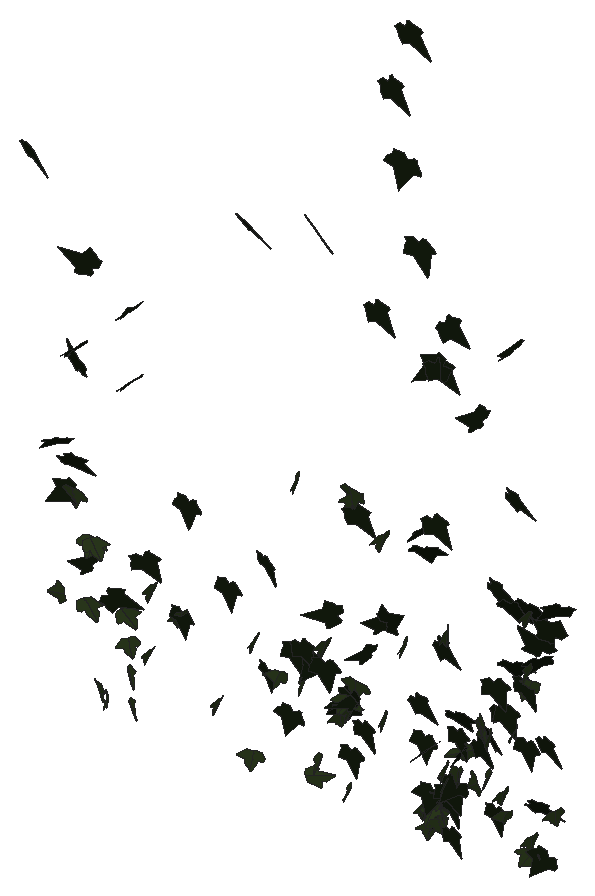
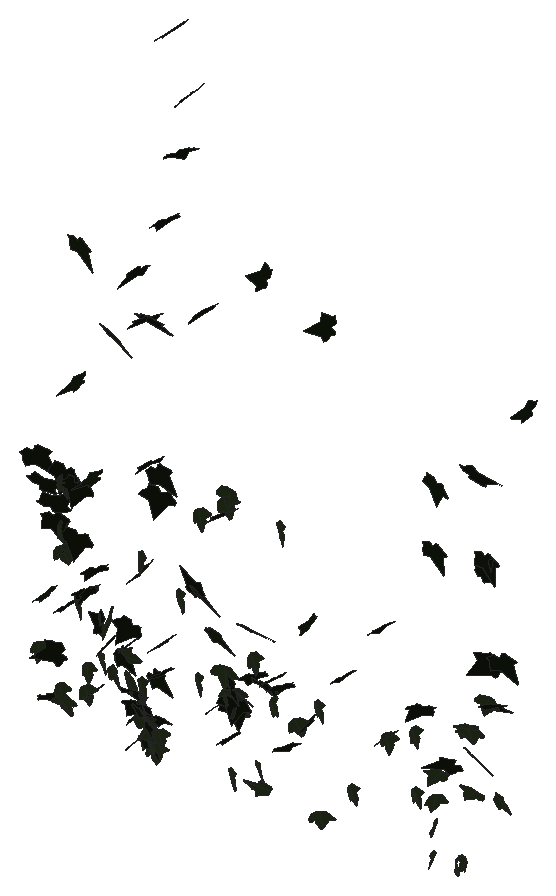
# SketchUp Ruby script. Lengths in inches.
U = 1.inch
M = Sketchup.active_model
def pt(a) = Geom::Point3d.new(a.map { |v| v * U })
def face(e, loops, mat)
  f = e.add_face(loops[0].map { |a| pt(a) })
  loops[1..].each { |l| e.add_face(l.map { |a| pt(a) }).erase! }
  f.material = f.back_material = mat if mat
  f
end
# faces: each face lists its corners as indices into pts; further lists are holes
def faces(e, pts, list, mat = nil) = list.each { |f| face(e, (f[0].is_a?(Array) ? f : [f]).map { |l| l.map { |i| pts[i] } }, mat) }
# xy, xz, yz: faces in a plane at the given z, y or x. An outline is a flat list of corners, or four numbers for a rectangle; further outlines are holes
def ring(l) = l.size == 4 ? [[l[0], l[1]], [l[2], l[1]], [l[2], l[3]], [l[0], l[3]]] : l.each_slice(2).to_a
def flat(e, list, mat, &to3) = list.each { |f| face(e, (f[0].is_a?(Array) ? f : [f]).map { |l| ring(l).map { |u, v| to3.(u, v) } }, mat) }
def xy(e, z, list, mat = nil) = flat(e, list, mat) { |x, y| [x, y, z] }
def xz(e, y, list, mat = nil) = flat(e, list, mat) { |x, z| [x, y, z] }
def yz(e, x, list, mat = nil) = flat(e, list, mat) { |y, z| [x, y, z] }
def lines(e, pts, list) = list.each { |a, b| e.add_line(pt(pts[a]), pt(pts[b])) }
# prism: a flat outline (further loops are holes) pulled along v
def prism(e, loops, v, mat = nil)
  f = face(e, loops, mat); d = Geom::Vector3d.new(v.map { |x| x * U })
  f.pushpull(f.normal.samedirection?(d) ? d.length : -d.length)
end
def box(e, o, s, mat = nil) = prism(e, [[o, [o[0] + s[0], o[1], o[2]], [o[0] + s[0], o[1] + s[1], o[2]], [o[0], o[1] + s[1], o[2]]]], [0, 0, s[2]], mat)
def at(x, y, z, deg = 0) = Geom::Transformation.translation(pt([x, y, z])) * Geom::Transformation.rotation(ORIGIN, Z_AXIS, deg.degrees)
def axes(o, x, y, z) = Geom::Transformation.new([*x, 0, *y, 0, *z, 0, *pt(o).to_a, 1])
def part(name) = M.definitions.add(name)
# library, detail: a bought-in or finely detailed component or shape, given as its bounding box
def library(name, o, s) = part(name).tap { |d| box(d.entities, o, s) }
def detail(e, o, s) = box(e.add_group.entities, o, s)
def put(e, d, t, mat = nil) = e.add_instance(d, t).tap { |i| i.material = mat if mat }
def group(e, t, mat = nil) = e.add_group.tap { |g| g.transformation = t; g.material = mat if mat }.entities
root = M.entities
M.materials.add("1026 AP 7946 SUNNY SIDE UP").color = [254, 231, 186]
M.materials.add("efeu1").color = [18, 25, 13]
M.materials.add("efeu2").color = [43, 57, 29]
c1 = part("ivyleaf_9")
p = [[1.54,2.16,1.25],[1.36,2.04,1.19],[-0.21,0.99,0.68],[-0.71,1.11,0.82],[-0.85,0.86,0.67],[-0.8,0.17,0.21],
  [-0.9,-0.01,0.1],[-0.67,-0.16,-0.02],[-0.08,-0.08,-0.05],[-0.03,-0.6,-0.4],[0.65,-0.88,-0.66],[0.83,-0.6,-0.49],
  [1.29,-0.42,-0.43],[1.8125,-0.07,-0.26],[1.21,0.44,0.15]]
faces(c1.entities,p,[[0,1,2,3,4,5,6,7,8,9,10,11,12,13,14]],"efeu1")
c2 = part("ivyleaf_10")
p = [[0,0.5,-0.03],[-0.0625,2.02,-0.43],[-0.19,2.01,-0.46],[-0.54,1.05,-0.29],[-0.52,0.625,-0.18],[-0.83,0.76,-0.28],
  [-1.16,0.64,-0.33],[-1.15,0.33,-0.24],[-0.77,-0.39,0.02],[-0.3,-0.51,0.16],[0.04,-0.48,0.23],[-0.02,2.01,-0.4375],
  [-0.06,2.01,-0.43],[0.04,-0.49,0.23],[0.67,-0.49,0.14],[1.38,0.36,-0.2],[1.375,0.51,-0.24],[0.81,0.65,-0.19],
  [0.62,0.59,-0.15],[0.6,1.09,-0.28],[0.5,1.23,-0.31]]
faces(c2.entities,p,[[0,1,2,3,4,5,6,7,8,9,10],[11,12,0,13,14,15,16,17,18,19,20]],"efeu2")
put(root,c1,axes([92.77,212.74,316.3125],[0.41895,-0.32591,0.01029],[-0.00018,-0.01746,-0.43776],[0.55374,0.24657,-0.00793]),"1026 AP 7946 SUNNY SIDE UP")
put(root,c1,axes([94.52,212.72,302.72],[-0.02841,0.30367,-0.19747],[-0.16541,-0.18535,-0.31314],[-0.58366,0.03775,0.09835]),"1026 AP 7946 SUNNY SIDE UP")
put(root,c2,axes([94.7,212.66,295.34],[-0.16673,0.10964,0.32224],[-0.51293,0.06853,-0.13195],[-0.17364,-0.30772,0.08038]),"1026 AP 7946 SUNNY SIDE UP")
put(root,c1,axes([94.97,213.07,300.27],[-0.48655,-0.13819,0.15485],[-0.18054,-0.1124,-0.33798],[0.29022,-0.3016,0.04934]),"1026 AP 7946 SUNNY SIDE UP")
put(root,c2,axes([95.21,212.84,300.38],[-0.58664,0.05585,-0.01158],[0.00571,-0.05082,-0.3717],[-0.09664,-0.34202,0.04833]),"1026 AP 7946 SUNNY SIDE UP")
put(root,c1,axes([95.52,212.57,307.59],[-0.06314,0.38301,-0.04846],[0.00462,-0.05023,-0.41267],[-0.65574,-0.03723,0.00176]),"1026 AP 7946 SUNNY SIDE UP")
put(root,c1,axes([95.16,212.49,302.15],[0.59339,0.07262,0.09594],[0.16097,-0.0234,-0.38002],[-0.10928,0.35987,-0.03882]),"1026 AP 7946 SUNNY SIDE UP")
put(root,c1,axes([95.68,212.59,306.68],[0.24493,-0.21206,0.30234],[-0.1526,0.27599,0.27227],[-0.58365,-0.16115,0.05569]),"1026 AP 7946 SUNNY SIDE UP")
put(root,c1,axes([96.24,212.68,311.73],[-0.21631,0.12586,0.37719],[-0.50429,0.18936,-0.18568],[-0.38172,-0.32149,0.03156]),"1026 AP 7946 SUNNY SIDE UP")
put(root,c1,axes([96.2,212.78,297.22],[-0.3481,0.24321,0.14613],[-0.18038,0.08427,-0.33836],[-0.4349,-0.22962,0.02337]),"1026 AP 7946 SUNNY SIDE UP")
put(root,c2,axes([95.97,212.77,295.27],[0.46366,0.09932,0.19462],[0.30964,0.02272,-0.30859],[-0.16255,0.32659,-0.03271]),"1026 AP 7946 SUNNY SIDE UP")
put(root,c2,axes([96.22,212.79,298.36],[0.5507,0.12241,-0.03423],[-0.02852,-0.0499,-0.36936],[-0.21358,0.3223,-0.03893]),"1026 AP 7946 SUNNY SIDE UP")
put(root,c2,axes([96.44,212.58,298.44],[0.34259,0.27024,0.10697],[0.14252,0.05707,-0.35868],[-0.46573,0.21625,-0.03107]),"1026 AP 7946 SUNNY SIDE UP")
put(root,c2,axes([96.6,212.8,291.5],[-0.33927,0.24106,-0.07943],[0.05341,-0.07412,-0.33541],[-0.42642,-0.20108,0.02119]),"1026 AP 7946 SUNNY SIDE UP")
put(root,c2,axes([97,212.84,290.94],[0.00194,0.03897,0.34568],[0.34533,-0.25137,0.02825],[0.42966,0.20186,-0.02426]),"1026 AP 7946 SUNNY SIDE UP")
put(root,c1,axes([97.41,212.61,296.17],[0.20133,-0.05882,-0.3478],[0.17778,0.33333,-0.01908],[0.53016,-0.08944,0.13848]),"1026 AP 7946 SUNNY SIDE UP")
put(root,c2,axes([98.06,212.74,295.5],[0.31669,0.23534,0.18952],[0.15023,0.15127,-0.31859],[-0.47353,0.20538,0.02567]),"1026 AP 7946 SUNNY SIDE UP")
put(root,c1,axes([98.47,212.46,310.37],[0.06266,0.35619,0.19543],[-0.02234,0.17966,-0.37967],[-0.67551,0.0271,0.03069]),"1026 AP 7946 SUNNY SIDE UP")
put(root,c2,axes([98.25,212.8,294.18],[-0.26313,-0.31714,-0.03009],[0.19509,-0.03647,-0.34591],[0.46094,-0.1656,0.12923]),"1026 AP 7946 SUNNY SIDE UP")
put(root,c1,axes([98.59,212.51,307.02],[-0.08154,0.38392,-0.02883],[-0.00118,-0.03227,-0.41464],[-0.65397,-0.04781,0.00434]),"1026 AP 7946 SUNNY SIDE UP")
put(root,c2,axes([98.32,212.76,292.77],[-0.1331,0.32518,-0.04013],[0.0039,-0.04236,-0.35861],[-0.55652,-0.07807,0.00708]),"1026 AP 7946 SUNNY SIDE UP")
put(root,c2,axes([98.38,212.81,291.15],[-0.21102,0.30309,0.03831],[-0.02924,0.02733,-0.35028],[-0.51651,-0.12538,0.00418]),"1026 AP 7946 SUNNY SIDE UP")
put(root,c1,axes([99.1,212.72,298.59],[-0.05917,-0.24061,-0.28203],[0.09695,0.25432,-0.25632],[0.59387,-0.06549,0.01375]),"1026 AP 7946 SUNNY SIDE UP")
put(root,c2,axes([99.39,212.84,294.09],[0.03169,-0.33777,0.02342],[-0.01919,-0.02693,-0.36228],[0.57479,0.01773,-0.01339]),"1026 AP 7946 SUNNY SIDE UP")
put(root,c2,axes([99.48,212.85,297.22],[0.00741,-0.36998,0.05555],[0.04253,-0.05554,-0.38056],[0.58685,0.00869,0.02688]),"1026 AP 7946 SUNNY SIDE UP")
put(root,c2,axes([101,212.87,296.43],[-0.13163,-0.35946,-0.02146],[0.00718,0.01823,-0.38011],[0.56594,-0.08383,-0.00017]),"1026 AP 7946 SUNNY SIDE UP")
put(root,c1,axes([101,212.96,296.4375],[0.00671,-0.36491,0.06415],[0.00484,-0.06431,-0.37632],[0.58261,0.00474,0.00239]),"1026 AP 7946 SUNNY SIDE UP")
put(root,c1,axes([101.41,212.88,302.01],[-0.07442,-0.3833,0.04911],[-0.0047,-0.04986,-0.39815],[0.60775,-0.04732,0.00294]),"1026 AP 7946 SUNNY SIDE UP")
put(root,c2,axes([103.0625,212.91,292.97],[0.05488,-0.3549,0.05585],[0.00156,-0.0564,-0.36768],[0.56501,0.03462,-0.00441]),"1026 AP 7946 SUNNY SIDE UP")
put(root,c1,axes([103.55,212.92,298.75],[-0.03552,-0.3778,0.01384],[-0.00328,-0.01549,-0.38999],[0.59455,-0.02266,-0.00132]),"1026 AP 7946 SUNNY SIDE UP")
put(root,c1,axes([104.29,212.92,316.7],[0.54739,-0.24082,0.11004],[0.12695,-0.07334,-0.43628],[0.39524,0.35709,-0.01227]),"1026 AP 7946 SUNNY SIDE UP")
put(root,c2,axes([104.9,212.89,291],[-0.42181,-0.22282,0.06068],[0.04131,-0.12113,-0.34218],[0.36055,-0.2468,0.11019]),"1026 AP 7946 SUNNY SIDE UP")
put(root,c2,axes([105.04,212.89,296.65],[0.11663,-0.36509,0.00197],[-0.00806,-0.00511,-0.38377],[0.57404,0.0741,-0.00579]),"1026 AP 7946 SUNNY SIDE UP")
put(root,c1,axes([105.54,212.88,300.7],[0.21894,-0.34894,0.09634],[0.02095,-0.09731,-0.38688],[0.56846,0.13798,-0.02284]),"1026 AP 7946 SUNNY SIDE UP")
put(root,c1,axes([105.71,212.88,295.35],[0.05988,-0.30921,0.20141],[0.04343,-0.19534,-0.32208],[0.57508,0.04695,0.00335]),"1026 AP 7946 SUNNY SIDE UP")
put(root,c2,axes([106.29,212.89,295.34],[-0.28626,-0.28488,0.15082],[0.00346,-0.17127,-0.33778],[0.50479,-0.16038,0.08784]),"1026 AP 7946 SUNNY SIDE UP")
put(root,c1,axes([107.06,212.86,293.8],[-0.22739,-0.33053,0.06427],[-0.0084,-0.06768,-0.37139],[0.52939,-0.14305,0.02171]),"1026 AP 7946 SUNNY SIDE UP")
put(root,c2,axes([107.27,212.88,305.21],[0.17004,-0.38362,-0.05972],[-0.00083,0.05777,-0.40997],[0.60955,0.10709,0.0161]),"1026 AP 7946 SUNNY SIDE UP")
put(root,c1,axes([107.17,212.91,296.95],[-0.06667,-0.35745,-0.11036],[0.03484,0.10317,-0.37009],[0.5848,-0.0469,0.00947]),"1026 AP 7946 SUNNY SIDE UP")
put(root,c2,axes([107.75,212.81,295.73],[0.1446,-0.31577,0.17879],[0.10975,-0.16199,-0.33919],[0.55723,0.11385,0.02041]),"1026 AP 7946 SUNNY SIDE UP")
put(root,c1,axes([107.54,212.86,297.26],[0.13078,-0.34814,-0.12081],[0.04322,0.1238,-0.36399],[0.57504,0.06987,0.05483]),"1026 AP 7946 SUNNY SIDE UP")
put(root,c1,axes([108.36,212.875,296.69],[-0.57143,-0.03796,-0.08856],[0.13951,-0.0281,-0.37473],[0.04773,-0.37233,0.0351]),"1026 AP 7946 SUNNY SIDE UP")
put(root,c1,axes([108.125,212.87,317.84],[0.362,-0.31008,0.21089],[0.1378,-0.19083,-0.39702],[0.56934,0.24335,-0.038]),"1026 AP 7946 SUNNY SIDE UP")
put(root,c2,axes([108.58,212.78,292.14],[0.30137,-0.30064,0.07127],[0.05337,-0.06242,-0.36763],[0.48275,0.19458,-0.00385]),"1026 AP 7946 SUNNY SIDE UP")
put(root,c2,axes([108.19,212.78,291.17],[0.16426,-0.02297,-0.35409],[0.53435,0.06486,0.10236],[0.08744,-0.35321,0.03967]),"1026 AP 7946 SUNNY SIDE UP")
put(root,c2,axes([108.86,212.83,297.8125],[-0.04985,-0.37922,0.0055],[0.00721,-0.0079,-0.39204],[0.59636,-0.0316,0.0052]),"1026 AP 7946 SUNNY SIDE UP")
put(root,c1,axes([109.37,212.89,299.29],[-0.50613,0.14778,0.15425],[-0.28154,-0.05143,-0.34648],[-0.17189,-0.35091,0.11328]),"1026 AP 7946 SUNNY SIDE UP")
put(root,c1,axes([108.93,212.74,296.85],[-0.13173,-0.354,-0.09943],[0.05376,0.08897,-0.37402],[0.57361,-0.08963,0.01222]),"1026 AP 7946 SUNNY SIDE UP")
put(root,c2,axes([109.73,212.76,294.68],[-0.16977,-0.34162,-0.10777],[0.06232,0.09511,-0.36843],[0.55742,-0.11468,0.00837]),"1026 AP 7946 SUNNY SIDE UP")
put(root,c1,axes([109.89,212.76,294.97],[0.24701,0.30377,-0.15371],[-0.06501,-0.14795,-0.35194],[-0.52938,0.15991,-0.0285]),"1026 AP 7946 SUNNY SIDE UP")
put(root,c1,axes([109.92,212.73,295.14],[0.34398,0.29354,-0.07906],[-0.05503,-0.07163,-0.37727],[-0.47456,0.22107,-0.01355]),"1026 AP 7946 SUNNY SIDE UP")
put(root,c2,axes([110.12,212.76,295.53],[0.50497,0.14716,-0.1305],[-0.2133,-0.00736,-0.36075],[-0.21966,0.34546,0.05029]),"1026 AP 7946 SUNNY SIDE UP")
put(root,c1,axes([110.39,212.72,295.72],[-0.55522,0.13201,0.0147],[-0.04542,-0.03895,-0.38561],[-0.20366,-0.35121,0.04592]),"1026 AP 7946 SUNNY SIDE UP")
put(root,c1,axes([110.43,212.76,296.1],[0.14819,-0.03219,-0.37553],[-0.57508,-0.00402,-0.09712],[0.00653,0.37631,-0.03094]),"1026 AP 7946 SUNNY SIDE UP")
put(root,c2,axes([110.23,212.71,291.24],[0.15806,-0.33878,-0.07248],[-0.04135,0.06356,-0.36361],[0.54189,0.10367,-0.0066]),"1026 AP 7946 SUNNY SIDE UP")
put(root,c2,axes([110.37,212.74,295.24],[0.02923,-0.37161,0.03654],[-0.00914,-0.0379,-0.38345],[0.58723,0.0179,-0.00779]),"1026 AP 7946 SUNNY SIDE UP")
put(root,c2,axes([110.43,212.87,305.42],[-0.20988,-0.3724,0.07701],[-0.00833,-0.07963,-0.40741],[0.59785,-0.13184,0.02136]),"1026 AP 7946 SUNNY SIDE UP")
put(root,c2,axes([110.44,212.65,305.81],[-0.58988,0.14518,0.03174],[-0.06174,-0.01865,-0.41325],[-0.22478,-0.37588,0.03023]),"1026 AP 7946 SUNNY SIDE UP")
put(root,c1,axes([110.33,212.77,293.1],[0.00001,-0.366,-0.02675],[-0.00423,0.02388,-0.3769],[0.57671,0.00018,-0.00276]),"1026 AP 7946 SUNNY SIDE UP")
put(root,c2,axes([110.64,212.74,296.49],[-0.58964,-0.01489,0.05691],[-0.08422,-0.03902,-0.38502],[0.032,-0.37704,0.03536]),"1026 AP 7946 SUNNY SIDE UP")
put(root,c1,axes([110.46,212.84,304.8125],[0.16476,-0.34622,-0.18059],[0.0711,0.18928,-0.36023],[0.60465,0.07208,0.09157]),"1026 AP 7946 SUNNY SIDE UP")
put(root,c1,axes([111.35,212.72,298.23],[-0.40581,0.28521,-0.01545],[-0.07269,-0.06379,-0.38861],[-0.44331,-0.25062,0.07786]),"1026 AP 7946 SUNNY SIDE UP")
put(root,c1,axes([110.96,212.77,294.5625],[0.13648,-0.35952,-0.04347],[-0.00011,0.04128,-0.38065],[0.56882,0.08627,0.01036]),"1026 AP 7946 SUNNY SIDE UP")
put(root,c1,axes([112.18,212.7,300.01],[-0.37732,0.29063,0.11044],[-0.14658,0.0594,-0.38646],[-0.46358,-0.25534,0.0323]),"1026 AP 7946 SUNNY SIDE UP")
put(root,c1,axes([111.55,212.87,315.07],[0.20184,-0.36833,-0.19172],[-0.03724,0.18583,-0.39912],[0.64634,0.12573,0.03688]),"1026 AP 7946 SUNNY SIDE UP")
put(root,c2,axes([112.08,212.71,304.17],[-0.08274,-0.39725,-0.01472],[0.01595,0.01079,-0.41266],[0.62471,-0.05289,0.00859]),"1026 AP 7946 SUNNY SIDE UP")
put(root,c2,axes([112.18,212.7,295.46],[0.16285,-0.35952,-0.00114],[0.03834,0.00606,-0.38453],[0.56401,0.10339,0.02647]),"1026 AP 7946 SUNNY SIDE UP")
put(root,c1,axes([112.24,212.73,300.02],[-0.09959,0.10626,0.38328],[0.30642,-0.31623,0.12558],[0.52455,0.2049,-0.00059]),"1026 AP 7946 SUNNY SIDE UP")
put(root,c1,axes([112.28,212.9,326.1875],[0.27091,-0.39526,-0.1743],[-0.06248,0.16443,-0.44234],[0.67177,0.17469,0.02915]),"1026 AP 7946 SUNNY SIDE UP")
put(root,c2,axes([113.3,212.66,299.4375],[0.16374,-0.37372,-0.02151],[0.00263,0.01993,-0.39949],[0.58838,0.10391,0.00777]),"1026 AP 7946 SUNNY SIDE UP")
put(root,c1,axes([113.19,212.91,322.71],[-0.27611,-0.41228,0.06238],[-0.00996,-0.06559,-0.46158],[0.65569,-0.17461,0.01925]),"1026 AP 7946 SUNNY SIDE UP")
put(root,c1,axes([113.25,212.9,329.19],[0.30524,-0.40528,-0.14743],[-0.00056,0.1544,-0.45741],[0.67463,0.1835,0.06633]),"1026 AP 7946 SUNNY SIDE UP")
put(root,c1,axes([113.9,212.89,318.94],[0.00461,-0.4356,-0.08502],[0.00844,0.08009,-0.44826],[0.69637,0.00191,0.006]),"1026 AP 7946 SUNNY SIDE UP")
put(root,c1,axes([113.93,212.71,296.89],[0.29967,-0.29146,-0.16248],[-0.04083,0.16638,-0.35181],[0.51825,0.18164,0.06624]),"1026 AP 7946 SUNNY SIDE UP")
put(root,c2,axes([114.35,212.74,291.88],[-0.05562,-0.35782,-0.01901],[0.01016,0.01586,-0.3703],[0.56314,-0.03563,0.0048]),"1026 AP 7946 SUNNY SIDE UP")
put(root,c1,axes([114.56,212.68,305.5],[-0.16494,0.32873,-0.22615],[-0.00568,-0.2298,-0.3511],[-0.62316,-0.08492,0.06306]),"1026 AP 7946 SUNNY SIDE UP")
put(root,c1,axes([114.35,212.68,304.39],[0.43691,0.28164,-0.09424],[-0.11287,-0.0599,-0.40783],[-0.45254,0.28685,0.01073]),"1026 AP 7946 SUNNY SIDE UP")
put(root,c1,axes([114.25,212.82,295.11],[-0.06172,-0.36873,0.01784],[0.00141,-0.01962,-0.38211],[0.58059,-0.03915,0.00283]),"1026 AP 7946 SUNNY SIDE UP")
put(root,c1,axes([114.66,212.74,294.82],[-0.26373,0.26738,-0.18747],[0.05813,-0.18947,-0.32035],[-0.50659,-0.16094,0.06084]),"1026 AP 7946 SUNNY SIDE UP")
put(root,c2,axes([114.65,212.75,291.02],[-0.2745,-0.30981,0.03402],[0.00627,-0.04208,-0.36575],[0.49016,-0.17296,0.02373]),"1026 AP 7946 SUNNY SIDE UP")
put(root,c2,axes([114.6875,212.87,291.81],[0.33109,0.2448,-0.15932],[-0.12505,-0.13676,-0.33236],[-0.43901,0.22357,-0.02549]),"1026 AP 7946 SUNNY SIDE UP")
put(root,c1,axes([114.68,212.83,292.69],[-0.43162,-0.20038,-0.12799],[0.2153,0.01766,-0.34404],[0.30064,-0.30032,0.06262]),"1026 AP 7946 SUNNY SIDE UP")
put(root,c2,axes([114.78,212.87,291.34],[0.17761,-0.32882,0.08228],[0.0204,-0.0819,-0.35837],[0.53238,0.11283,-0.01372]),"1026 AP 7946 SUNNY SIDE UP")
put(root,c1,axes([115.13,212.89,313.42],[-0.67342,0.00145,0.03076],[-0.04693,-0.04373,-0.43916],[0.00252,-0.42708,0.04255]),"1026 AP 7946 SUNNY SIDE UP")
put(root,c1,axes([114.95,212.87,292.3125],[-0.3071,0.12701,-0.28183],[0.28084,-0.21496,-0.23482],[-0.38344,-0.25917,0.05373]),"1026 AP 7946 SUNNY SIDE UP")
put(root,c1,axes([115.11,212.8,291.41],[-0.25788,0.30286,-0.08219],[0.0514,-0.07496,-0.35518],[-0.49047,-0.16709,0.00599]),"1026 AP 7946 SUNNY SIDE UP")
put(root,c2,axes([115.28,212.85,292.38],[-0.38653,-0.06785,0.2617],[-0.33156,-0.15772,-0.25415],[0.24796,-0.31667,0.06811]),"1026 AP 7946 SUNNY SIDE UP")
put(root,c1,axes([114.83,212.71,305.91],[0.14045,-0.36138,-0.18071],[0.0113,0.17903,-0.37961],[0.63014,0.07734,0.04708]),"1026 AP 7946 SUNNY SIDE UP")
put(root,c2,axes([115.14,212.62,291.5],[-0.21542,-0.31597,-0.10444],[0.14074,0.06846,-0.35021],[0.50155,-0.15492,0.05341]),"1026 AP 7946 SUNNY SIDE UP")
put(root,c2,axes([115.25,212.83,292.65],[0.35445,-0.27832,0.03724],[0.00533,-0.04567,-0.36827],[0.4416,0.22395,-0.02544]),"1026 AP 7946 SUNNY SIDE UP")
put(root,c1,axes([114.93,212.8125,313.45],[0.15965,-0.363,-0.21812],[0.07881,0.22469,-0.37445],[0.65443,0.0615,0.09831]),"1026 AP 7946 SUNNY SIDE UP")
put(root,c2,axes([115.2,212.86,291.86],[-0.11079,0.33823,-0.10063],[0.03192,-0.09752,-0.3565],[-0.5535,-0.07332,-0.00041]),"1026 AP 7946 SUNNY SIDE UP")
put(root,c1,axes([115.61,212.76,292.875],[-0.3385,0.28051,-0.08545],[0.02007,-0.09583,-0.36161],[-0.46023,-0.21049,0.04708]),"1026 AP 7946 SUNNY SIDE UP")
put(root,c2,axes([115.38,212.8125,293.38],[0.21551,-0.33975,-0.01489],[0.00859,0.01571,-0.37715],[0.53452,0.13673,0.01207]),"1026 AP 7946 SUNNY SIDE UP")
put(root,c2,axes([115.46,212.74,294.13],[0.1261,-0.38431,-0.00996],[0.00452,0.00825,-0.40436],[0.60438,0.08012,0.0051]),"1026 AP 7946 SUNNY SIDE UP")
put(root,c2,axes([115.5,212.73,300.71],[0.11874,-0.37456,-0.09744],[0.06777,0.10181,-0.38805],[0.60284,0.06233,0.06281]),"1026 AP 7946 SUNNY SIDE UP")
put(root,c1,axes([115.29,212.56,300.16],[0.36099,-0.27575,-0.20747],[-0.14028,0.18387,-0.36592],[0.51676,0.24254,0.04559]),"1026 AP 7946 SUNNY SIDE UP")
put(root,c1,axes([115.52,212.9,293.03],[-0.25079,-0.18681,-0.27384],[0.31687,0.17389,-0.25045],[0.39898,-0.25553,0.02678]),"1026 AP 7946 SUNNY SIDE UP")
put(root,c1,axes([115.55,212.73,315.7],[0.21493,-0.26476,-0.33027],[-0.11935,0.31433,-0.30034],[0.64095,0.14731,0.05483]),"1026 AP 7946 SUNNY SIDE UP")
put(root,c1,axes([115.6,212.9,292.43],[0.12409,-0.34957,0.02742],[-0.00851,-0.03053,-0.36916],[0.55143,0.0782,-0.01187]),"1026 AP 7946 SUNNY SIDE UP")
put(root,c1,axes([115.68,212.79,291.0625],[0.15763,-0.33575,-0.059],[-0.03885,0.05039,-0.36056],[0.53366,0.10284,-0.00882]),"1026 AP 7946 SUNNY SIDE UP")
put(root,c1,axes([116.1,212.8,293.55],[-0.54764,-0.0998,-0.0421],[0.07505,-0.02087,-0.37181],[0.15169,-0.34999,0.03196]),"1026 AP 7946 SUNNY SIDE UP")
put(root,c2,axes([116.05,212.71,294.09],[0.3943,-0.27324,0.00747],[0.10333,0.04865,-0.37249],[0.41727,0.24615,0.08518]),"1026 AP 7946 SUNNY SIDE UP")
put(root,c1,axes([116.05,212.72,296.91],[0.55421,0.10753,-0.05586],[-0.07725,-0.0268,-0.37961],[-0.17337,0.35569,-0.00943]),"1026 AP 7946 SUNNY SIDE UP")
put(root,c2,axes([116.53,212.85,295.27],[-0.13195,-0.09244,0.35816],[-0.29257,-0.29501,-0.12861],[0.48505,-0.20309,0.01986]),"1026 AP 7946 SUNNY SIDE UP")
put(root,c2,axes([116.27,212.72,294.14],[0.24686,-0.33185,-0.02947],[0.01284,0.03338,-0.37734],[0.52333,0.15572,0.02316]),"1026 AP 7946 SUNNY SIDE UP")
put(root,c1,axes([116.07,212.8,295.99],[0.11693,-0.3681,-0.02968],[-0.02703,0.02377,-0.38653],[0.57969,0.07535,-0.01203]),"1026 AP 7946 SUNNY SIDE UP")
put(root,c1,axes([116.53,212.82,295.37],[-0.20114,0.274,-0.21841],[0.13304,-0.19616,-0.31262],[-0.52981,-0.15328,0.00442]),"1026 AP 7946 SUNNY SIDE UP")
put(root,c2,axes([117.29,212.53,294.07],[-0.28685,0.15513,0.29599],[-0.43002,0.10542,-0.23763],[-0.27827,-0.32281,0.06211]),"1026 AP 7946 SUNNY SIDE UP")
put(root,c1,axes([117.44,212.62,311.74],[-0.38165,0.32012,0.15816],[-0.18501,0.10061,-0.41205],[-0.52539,-0.26796,0.03021]),"1026 AP 7946 SUNNY SIDE UP")
put(root,c1,axes([117.14,212.85,295.82],[0.25129,-0.28596,-0.18335],[-0.13994,0.15228,-0.33657],[0.5094,0.1829,-0.00201]),"1026 AP 7946 SUNNY SIDE UP")
put(root,c2,axes([117.3,212.87,296.66],[-0.18023,0.2812,0.22759],[0.16265,-0.19425,0.31113],[0.53663,0.15332,-0.01787]),"1026 AP 7946 SUNNY SIDE UP")
put(root,c2,axes([117.37,212.85,296.48],[-0.18199,0.35625,-0.01043],[-0.0132,-0.0155,-0.38576],[-0.56034,-0.11534,0.01248]),"1026 AP 7946 SUNNY SIDE UP")
put(root,c2,axes([117.83,212.71,294.6],[0.23524,-0.33767,0.00077],[-0.00742,-0.00501,-0.38045],[0.53091,0.14955,-0.00566]),"1026 AP 7946 SUNNY SIDE UP")
put(root,c2,axes([117.88,212.67,296.57],[0.18226,-0.34955,-0.05512],[0.01402,0.0571,-0.37809],[0.55539,0.11327,0.02763]),"1026 AP 7946 SUNNY SIDE UP")
put(root,c1,axes([117.74,212.81,296.48],[0.2274,-0.0648,-0.35144],[0.52156,-0.08221,0.16064],[-0.15962,-0.36095,0.02422]),"1026 AP 7946 SUNNY SIDE UP")
put(root,c1,axes([118.02,212.9375,292.89],[0.05173,-0.35681,0.02956],[-0.00201,-0.03097,-0.3693],[0.56312,0.03267,-0.00403]),"1026 AP 7946 SUNNY SIDE UP")
put(root,c1,axes([118.13,212.71,299.15],[-0.01797,-0.34703,-0.16473],[0.03524,0.15711,-0.35642],[0.59849,-0.01967,0.01604]),"1026 AP 7946 SUNNY SIDE UP")
put(root,c1,axes([118.125,212.67,303.91],[0.47747,-0.22976,-0.14326],[-0.0539,0.17319,-0.37442],[0.41778,0.28494,0.11542]),"1026 AP 7946 SUNNY SIDE UP")
put(root,c2,axes([118.51,212.95,292.8125],[-0.15955,-0.33996,0.05361],[-0.00395,-0.05553,-0.36556],[0.54123,-0.10062,0.01313]),"1026 AP 7946 SUNNY SIDE UP")
put(root,c2,axes([118.5,212.83,293.93],[-0.05799,-0.35768,-0.07426],[0.01106,0.0697,-0.37003],[0.573,-0.03755,-0.00037]),"1026 AP 7946 SUNNY SIDE UP")
put(root,c1,axes([118.36,212.77,298.02],[0.14873,-0.27427,-0.25314],[-0.13736,0.22809,-0.29748],[0.56082,0.1286,-0.00573]),"1026 AP 7946 SUNNY SIDE UP")
put(root,c1,axes([118.59,212.82,297.94],[-0.0024,-0.35194,-0.15324],[0.03116,0.14648,-0.36125],[0.59877,-0.00904,0.01819]),"1026 AP 7946 SUNNY SIDE UP")
put(root,c1,axes([119.21,212.61,315.78],[-0.21783,0.4185,0.03006],[-0.03772,0.02027,-0.45371],[-0.65832,-0.13964,0.01606]),"1026 AP 7946 SUNNY SIDE UP")
put(root,c1,axes([119,212.76,303.28],[0.52011,0.16527,-0.13814],[-0.16581,-0.08997,-0.38009],[-0.29176,0.34576,-0.03024]),"1026 AP 7946 SUNNY SIDE UP")
put(root,c2,axes([119.13,212.82,297.18],[0.16582,-0.3514,-0.09837],[-0.04924,0.08821,-0.37742],[0.56964,0.10992,-0.00399]),"1026 AP 7946 SUNNY SIDE UP")
put(root,c1,axes([119.18,212.68,300.49],[0.44488,0.23194,-0.14509],[-0.18004,-0.08451,-0.37733],[-0.38802,0.30515,0.00873]),"1026 AP 7946 SUNNY SIDE UP")
put(root,c1,axes([119.06,212.66,308.62],[0.49105,-0.23748,-0.15372],[-0.10221,0.15394,-0.39524],[0.42785,0.30934,0.08201]),"1026 AP 7946 SUNNY SIDE UP")
put(root,c2,axes([119.9,212.94,299.62],[-0.30984,-0.2874,0.15897],[-0.02562,-0.17321,-0.3511],[0.51351,-0.18206,0.0784]),"1026 AP 7946 SUNNY SIDE UP")
put(root,c1,axes([119.65,212.81,299.72],[0.12529,-0.37506,-0.05943],[0.00021,0.0568,-0.39449],[0.59619,0.0788,0.01262]),"1026 AP 7946 SUNNY SIDE UP")
put(root,c2,axes([119.99,212.82,303.18],[-0.00332,-0.39777,0.02287],[-0.02319,-0.02437,-0.40965],[0.62621,-0.00301,-0.01505]),"1026 AP 7946 SUNNY SIDE UP")
put(root,c1,axes([119.76,212.87,296.72],[-0.00148,-0.37502,0.00879],[-0.00022,-0.01066,-0.38641],[0.58993,-0.00095,-0.00012]),"1026 AP 7946 SUNNY SIDE UP")
put(root,c1,axes([119.96,212.625,303.62],[0.51977,0.09137,-0.20257],[-0.28719,-0.07761,-0.35299],[-0.1851,0.37698,-0.02115]),"1026 AP 7946 SUNNY SIDE UP")
put(root,c2,axes([120.13,212.63,291.59],[0.53074,-0.01514,-0.13876],[-0.20827,0.03877,-0.34643],[0.04458,0.36131,0.0335]),"1026 AP 7946 SUNNY SIDE UP")
put(root,c2,axes([120.05,212.8,300.61],[0.10889,-0.34197,0.17754],[0.04583,-0.17189,-0.36041],[0.60177,0.07497,-0.00467]),"1026 AP 7946 SUNNY SIDE UP")
put(root,c2,axes([120.1,212.78,292.29],[-0.08047,-0.35125,-0.05297],[0.04111,0.04607,-0.36488],[0.55623,-0.05422,0.01931]),"1026 AP 7946 SUNNY SIDE UP")
put(root,c1,axes([120.6,212.79,301.62],[0.19308,0.03944,0.38379],[-0.58375,0.06353,0.11958],[-0.07618,-0.38686,0.05642]),"1026 AP 7946 SUNNY SIDE UP")
put(root,c1,axes([120.47,212.79,301.0625],[0.05132,0.33545,-0.20364],[-0.02467,-0.19898,-0.34836],[-0.61326,0.03607,-0.00303]),"1026 AP 7946 SUNNY SIDE UP")
put(root,c1,axes([120.24,212.7,294],[0.52829,-0.00046,0.16731],[0.25517,-0.01363,-0.34598],[0.00998,0.37292,-0.01025]),"1026 AP 7946 SUNNY SIDE UP")
put(root,c1,axes([120.85,212.84,291.63],[-0.40841,-0.23824,0.06522],[-0.05199,-0.05944,-0.36279],[0.38467,-0.26098,0.02021]),"1026 AP 7946 SUNNY SIDE UP")
put(root,c1,axes([121.25,212.82,302.52],[0.02812,0.07504,0.40108],[-0.54139,0.19537,-0.02138],[-0.30783,-0.33674,0.07424]),"1026 AP 7946 SUNNY SIDE UP")
put(root,c1,axes([120.64,212.9375,297.11],[0.28595,-0.32275,-0.05766],[-0.00242,0.06109,-0.38016],[0.51457,0.17964,0.03025]),"1026 AP 7946 SUNNY SIDE UP")
put(root,c2,axes([121.4,212.74,293.99],[-0.18194,-0.33531,-0.08857],[0.07057,0.07334,-0.36452],[0.53895,-0.12279,0.01783]),"1026 AP 7946 SUNNY SIDE UP")
put(root,c1,axes([121.68,212.73,304.04],[-0.02078,0.25569,-0.31567],[-0.17145,-0.29868,-0.25248],[-0.60547,0.0758,0.08233]),"1026 AP 7946 SUNNY SIDE UP")
